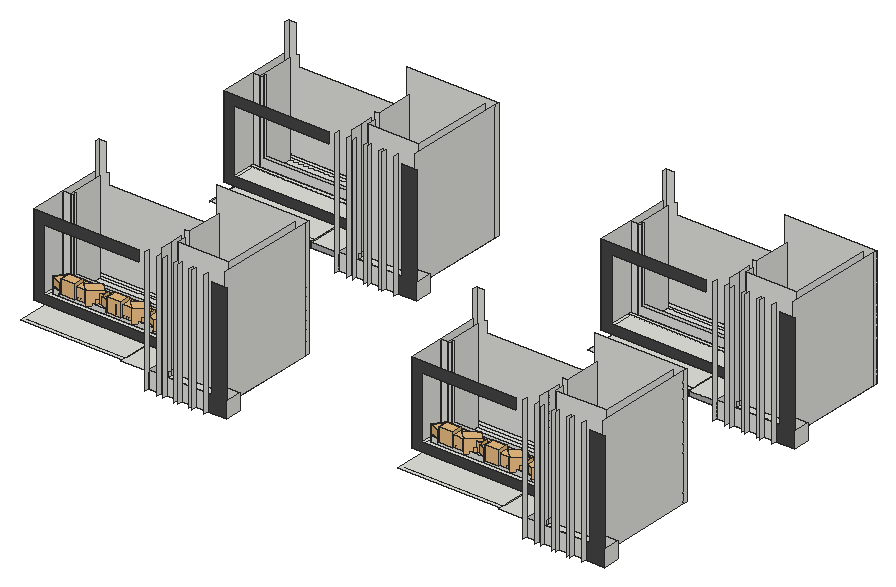
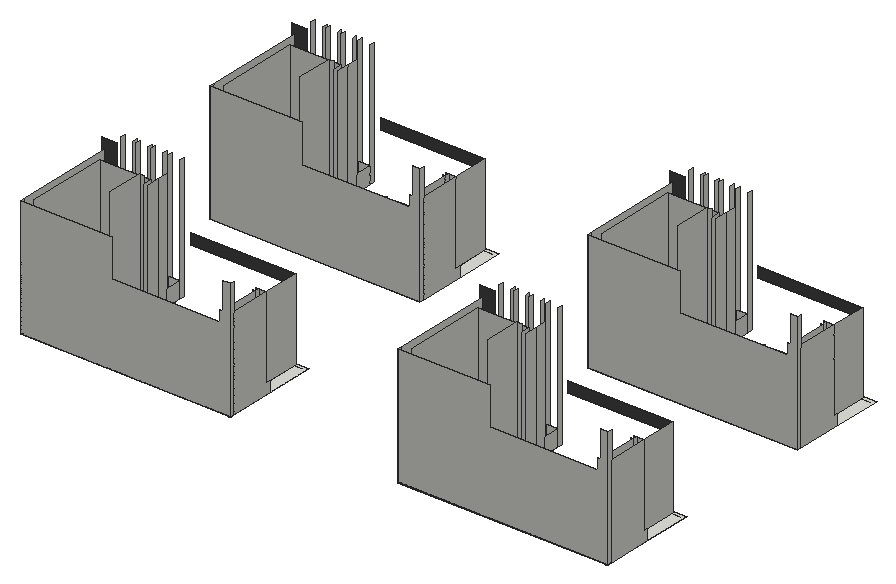
# SketchUp Ruby script. Lengths in inches.
U = 1.inch
M = Sketchup.active_model
def pt(a) = Geom::Point3d.new(a.map { |v| v * U })
def face(e, loops, mat)
  f = e.add_face(loops[0].map { |a| pt(a) })
  loops[1..].each { |l| e.add_face(l.map { |a| pt(a) }).erase! }
  f.material = f.back_material = mat if mat
  f
end
# faces: each face lists its corners as indices into pts; further lists are holes
def faces(e, pts, list, mat = nil) = list.each { |f| face(e, (f[0].is_a?(Array) ? f : [f]).map { |l| l.map { |i| pts[i] } }, mat) }
# xy, xz, yz: faces in a plane at the given z, y or x. An outline is a flat list of corners, or four numbers for a rectangle; further outlines are holes
def ring(l) = l.size == 4 ? [[l[0], l[1]], [l[2], l[1]], [l[2], l[3]], [l[0], l[3]]] : l.each_slice(2).to_a
def flat(e, list, mat, &to3) = list.each { |f| face(e, (f[0].is_a?(Array) ? f : [f]).map { |l| ring(l).map { |u, v| to3.(u, v) } }, mat) }
def xy(e, z, list, mat = nil) = flat(e, list, mat) { |x, y| [x, y, z] }
def xz(e, y, list, mat = nil) = flat(e, list, mat) { |x, z| [x, y, z] }
def yz(e, x, list, mat = nil) = flat(e, list, mat) { |y, z| [x, y, z] }
def lines(e, pts, list) = list.each { |a, b| e.add_line(pt(pts[a]), pt(pts[b])) }
# prism: a flat outline (further loops are holes) pulled along v
def prism(e, loops, v, mat = nil)
  f = face(e, loops, mat); d = Geom::Vector3d.new(v.map { |x| x * U })
  f.pushpull(f.normal.samedirection?(d) ? d.length : -d.length)
end
def box(e, o, s, mat = nil) = prism(e, [[o, [o[0] + s[0], o[1], o[2]], [o[0] + s[0], o[1] + s[1], o[2]], [o[0], o[1] + s[1], o[2]]]], [0, 0, s[2]], mat)
def at(x, y, z, deg = 0) = Geom::Transformation.translation(pt([x, y, z])) * Geom::Transformation.rotation(ORIGIN, Z_AXIS, deg.degrees)
def axes(o, x, y, z) = Geom::Transformation.new([*x, 0, *y, 0, *z, 0, *pt(o).to_a, 1])
def part(name) = M.definitions.add(name)
# library, detail: a bought-in or finely detailed component or shape, given as its bounding box
def library(name, o, s) = part(name).tap { |d| box(d.entities, o, s) }
def detail(e, o, s) = box(e.add_group.entities, o, s)
def put(e, d, t, mat = nil) = e.add_instance(d, t).tap { |i| i.material = mat if mat }
def group(e, t, mat = nil) = e.add_group.tap { |g| g.transformation = t; g.material = mat if mat }.entities
root = M.entities
M.materials.add("Material__1").color = [95, 70, 46]
M.materials.add("[Color M03]1").color = [170, 170, 170]
M.materials.add("[Granite Dark Gray]").color = [69, 68, 68]
c1 = library("Areca palm plant",[0,0,0],[49.1,36.6,54.46])
c2 = library("Group\#589",[-84.69,-90.07,-0.36],[176.51,175.13,171.4])
c3 = library("Group20\#1",[-20.81,-17.08,3.79],[39.86,39.43,37.51])
c4 = library("Group38\#1",[14.01,28.44,-23.43],[18.58,18.32,38.89])
c5 = library("Group\#590",[-7.34,-1.2,0],[38.67,35.81,49.04])
c6 = part("Group\#592")
put(c6.entities,c1,axes([-6.2,56.6,6.08],[0.45017,-0.56191,0],[0.66137,0.52986,0],[0,0,0.72]))
put(c6.entities,c1,axes([-6.2,158.41,6.08],[0.45017,-0.56191,0],[0.66137,0.52986,0],[0,0,0.72]))
put(c6.entities,c2,axes([17.19,15.79,6.07],[-0.08133,-0.14087,0],[0.14087,-0.08133,0],[0,0,0.1725]))
put(c6.entities,c3,axes([18.97,79.98,4.77],[0,0.85,0],[-0.85,0,0],[0,0,0.85]))
put(c6.entities,c4,axes([-4.1,-1.15,28.17],[0.8848,0,0],[0,0.94674,0],[0,0,0.85826]))
put(c6.entities,c2,axes([17.19,121.23,6.07],[-0.08133,-0.14087,0],[0.14087,-0.08133,0],[0,0,0.1725]))
put(c6.entities,c2,axes([14.93,91.37,6.05],[-0.04961,-0.08593,0],[0.08593,-0.04961,0],[0,0,0.10522]))
put(c6.entities,c3,axes([18.97,181.79,4.77],[0,0.85,0],[-0.85,0,0],[0,0,0.85]))
put(c6.entities,c2,axes([14.93,193.18,6.05],[-0.04961,-0.08593,0],[0.08593,-0.04961,0],[0,0,0.10522]))
put(c6.entities,c4,axes([-4.1,100.66,28.17],[0.8848,0,0],[0,0.94674,0],[0,0,0.85826]))
g1 = group(c6.entities,at(0,0,0))
xy(g1,0,[[0,0,6,234.8],[30,0,36,234.8]])
xy(g1,3,[[6,0,30,234.8]])
xy(g1,7,[[6,5,30,229.8]],"Material__1")
xy(g1,15,[[[0,0,36,234.8],[6,5,30,229.8]]])
xz(g1,0,[[0,0,6,0,6,3,30,3,30,0,36,0,36,15,0,15]])
xz(g1,5,[[6,7,30,15]])
xz(g1,229.8,[[6,7,30,15]])
xz(g1,234.8,[[0,0,0,15,36,15,36,0,30,0,30,3,6,3,6,0]])
yz(g1,0,[[0,0,234.8,15]])
yz(g1,6,[[0,0,234.8,3],[5,7,229.8,15]])
yz(g1,30,[[0,0,234.8,3],[5,7,229.8,15]])
yz(g1,36,[[0,0,234.8,15]])
put(c6.entities,c2,axes([17.19,223.04,6.07],[-0.08133,-0.14087,0],[0.14087,-0.08133,0],[0,0,0.1725]))
put(c6.entities,c2,axes([14.93,44.05,6.05],[-0.04961,-0.08593,0],[0.08593,-0.04961,0],[0,0,0.10522]))
put(c6.entities,c2,axes([14.93,173.12,6.05],[-0.04961,-0.08593,0],[0.08593,-0.04961,0],[0,0,0.10522]))
put(c6.entities,c2,axes([14.93,145.87,6.05],[-0.04961,-0.08593,0],[0.08593,-0.04961,0],[0,0,0.10522]))
put(c6.entities,c5,axes([24.9375,89.91,8],[0,0.79,0],[-0.79,0,0],[0,0,0.79]))
put(c6.entities,c2,axes([14.93,71.3,6.05],[-0.04961,-0.08593,0],[0.08593,-0.04961,0],[0,0,0.10522]))
put(c6.entities,c5,axes([24.9375,191.72,8],[0,0.79,0],[-0.79,0,0],[0,0,0.79]))
xy(root,144.9375,[[609.34,322.97,609.34,341.03,626.68,341.03,626.68,368.59,641.55,368.59,641.55,322.97],[641.55,322.97,657.03,387.84],[657.03,322.97,689.24,368.59],[689.24,322.97,698.65,387.84],[698.65,322.97,730.86,368.59],
  [730.86,322.97,739.28,387.84],[739.28,322.97,771.49,368.59],[771.49,322.97,771.49,387.84,782.78,387.84,782.78,368.59,824.53,368.59,824.53,322.97],[1657.65,322.97,1657.65,341.03,1674.99,341.03,1674.99,368.59,1689.86,368.59,1689.86,322.97],[1689.86,322.97,1705.34,387.84],
  [1705.34,322.97,1737.55,368.59],[1737.55,322.97,1746.96,387.84],[1746.96,322.97,1779.17,368.59],[1779.17,322.97,1787.59,387.84],[1787.59,322.97,1819.8,368.59],
  [1819.8,322.97,1819.8,387.84,1831.09,387.84,1831.09,368.59,1872.84,368.59,1872.84,322.97],[609.09,341.03,609.34,365.47],[609.34,341.03,626.68,365.47],[1657.41,341.03,1657.65,365.47],[1657.65,341.03,1674.99,365.47],
  [609.09,365.47,609.34,387.84],[609.34,365.47,626.68,368.59],[1657.41,365.47,1657.65,387.84],[1657.65,365.47,1674.99,368.59],[609.34,368.59,626.68,387.84],
  [626.68,368.59,641.55,387.84],[657.03,368.59,689.24,387.84],[698.65,368.59,730.86,387.84],[739.28,368.59,771.49,387.84],[1657.65,368.59,1674.99,387.84],
  [1674.99,368.59,1689.86,387.84],[1705.34,368.59,1737.55,387.84],[1746.96,368.59,1779.17,387.84],[1787.59,368.59,1819.8,387.84],[200.03,387.84,497.6,523.47],
  [[626.68,387.84,626.68,389.4,609.34,389.4,609.34,523.47,200.03,523.47,200.03,647.98,782.78,647.98,782.78,387.84],[620.86,408.96,761.66,408.96,761.66,637.97,221.15,637.97,221.15,534.98,620.86,534.98]],[609.09,387.84,609.34,389.4],[609.34,387.84,626.68,389.4],[1248.34,387.84,1545.92,523.47],[[1674.99,387.84,1674.99,389.4,1657.65,389.4,1657.65,523.47,1248.34,523.47,1248.34,647.98,1831.09,647.98,1831.09,387.84],[1669.17,408.96,1809.97,408.96,1809.97,637.97,1269.46,637.97,1269.46,534.98,1669.17,534.98]],
  [1657.41,387.84,1657.65,389.4],[1657.65,387.84,1674.99,389.4],[620.86,408.96,761.66,408.96,761.66,637.97,221.15,637.97,221.15,534.98,620.86,534.98],[1669.17,408.96,1809.97,408.96,1809.97,637.97,1269.46,637.97,1269.46,534.98,1669.17,534.98],[200.03,647.98,782.78,659.09],
  [1248.34,647.98,1831.09,659.09]])
xy(root,148.75,[[497.26,1024.56,497.26,1046.93,499.1875,1046.93,499.1875,1136.18,608.75,1136.18,608.75,1024.56],[608.75,1024.56,626.34,1046.93],[1545.57,1024.56,1545.57,1046.93,1547.5,1046.93,1547.5,1136.18,1657.0625,1136.18,1657.0625,1024.56],[1657.0625,1024.56,1674.65,1046.93],[608.75,1046.93,626.34,1046.93,626.34,1054,616.11,1054,616.11,1136.18,608.75,1136.18],
  [1657.0625,1046.93,1674.65,1046.93,1674.65,1054,1664.42,1054,1664.42,1136.18,1657.0625,1136.18],[616.11,1054,626.34,1136.18],[1664.42,1054,1674.65,1136.18],[607.28,1136.18,616.11,1153.68],[1655.6,1136.18,1664.42,1153.68]])
xy(root,149.375,[[609,982.06,609,1000.12,626.34,1000.12,626.34,1027.68,641.2,1027.68,641.2,982.06],[641.2,982.06,656.68,1046.93],[656.68,982.06,688.89,1027.68],[688.89,982.06,698.31,1046.93],[698.31,982.06,730.52,1027.68],
  [730.52,982.06,738.93,1046.93],[738.93,982.06,771.14,1027.68],[771.14,982.06,771.14,1046.93,782.4375,1046.93,782.4375,1027.68,824.1875,1027.68,824.1875,982.06],[1657.31,982.06,1657.31,1000.12,1674.65,1000.12,1674.65,1027.68,1689.52,1027.68,1689.52,982.06],[1689.52,982.06,1705,1046.93],
  [1705,982.06,1737.2,1027.68],[1737.2,982.06,1746.62,1046.93],[1746.62,982.06,1778.83,1027.68],[1778.83,982.06,1787.25,1046.93],[1787.25,982.06,1819.45,1027.68],
  [1819.45,982.06,1819.45,1046.93,1830.75,1046.93,1830.75,1027.68,1872.5,1027.68,1872.5,982.06],[608.75,1000.12,609,1024.56],[609,1000.12,626.34,1024.56],[1657.0625,1000.12,1657.31,1024.56],[1657.31,1000.12,1674.65,1024.56],
  [608.75,1024.56,609,1046.93],[609,1024.56,626.34,1027.68],[1657.0625,1024.56,1657.31,1046.93],[1657.31,1024.56,1674.65,1027.68],[609,1027.68,626.34,1046.93],
  [626.34,1027.68,641.2,1046.93],[656.68,1027.68,688.89,1046.93],[698.31,1027.68,730.52,1046.93],[738.93,1027.68,771.14,1046.93],[1657.31,1027.68,1674.65,1046.93],
  [1674.65,1027.68,1689.52,1046.93],[1705,1027.68,1737.2,1046.93],[1746.62,1027.68,1778.83,1046.93],[1787.25,1027.68,1819.45,1046.93],[199.6875,1046.93,497.26,1182.56],
  [[626.34,1046.93,626.34,1048.49,609,1048.49,609,1182.56,199.6875,1182.56,199.6875,1307.07,782.4375,1307.07,782.4375,1046.93],[620.51,1068.05,761.32,1068.05,761.32,1297.06,220.81,1297.06,220.81,1194.07,620.51,1194.07]],[608.75,1046.93,609,1048.49],[609,1046.93,626.34,1048.49],[1248,1046.93,1545.57,1182.56],[[1674.65,1046.93,1674.65,1048.49,1657.31,1048.49,1657.31,1182.56,1248,1182.56,1248,1307.07,1830.75,1307.07,1830.75,1046.93],[1668.82,1068.05,1809.63,1068.05,1809.63,1297.06,1269.12,1297.06,1269.12,1194.07,1668.82,1194.07]],
  [1657.0625,1046.93,1657.31,1048.49],[1657.31,1046.93,1674.65,1048.49],[620.51,1068.05,761.32,1068.05,761.32,1297.06,220.81,1297.06,220.81,1194.07,620.51,1194.07],[1668.82,1068.05,1809.63,1068.05,1809.63,1297.06,1269.12,1297.06,1269.12,1194.07,1668.82,1194.07],[199.6875,1307.07,782.4375,1318.18],
  [1248,1307.07,1830.75,1318.18]])
xy(root,157.5,[[497.6,365.47,609.09,365.47,609.09,387.84,609.34,387.84,609.34,523.47,497.6,523.47],[1545.92,365.47,1657.41,365.47,1657.41,387.84,1657.65,387.84,1657.65,523.47,1545.92,523.47]])
xy(root,161.9375,[[497.26,1024.56,608.75,1024.56,608.75,1046.93,609,1046.93,609,1182.56,497.26,1182.56],[1545.57,1024.56,1657.0625,1024.56,1657.0625,1046.93,1657.31,1046.93,1657.31,1182.56,1545.57,1182.56]])
xy(root,174.125,[[200.03,433.78,209.64,523.47],[609.34,433.78,609.34,523.47,200.03,523.47,200.03,534.98,620.86,534.98,620.86,433.78],[209.64,433.78,609.34,523.47],[620.86,433.78,632.79,534.98],[1248.34,433.78,1257.95,523.47],
  [1657.65,433.78,1657.65,523.47,1248.34,523.47,1248.34,534.98,1669.17,534.98,1669.17,433.78],[1257.95,433.78,1657.65,523.47],[1669.17,433.78,1681.11,534.98],[221.15,534.98,620.86,546.92],[620.86,534.98,632.79,546.92],
  [1269.46,534.98,1669.17,546.92],[1669.17,534.98,1681.11,546.92]])
xy(root,178.5625,[[199.6875,1092.87,209.29,1182.56],[609,1092.87,609,1182.56,199.6875,1182.56,199.6875,1194.07,620.51,1194.07,620.51,1092.87],[209.29,1092.87,609,1182.56],[620.51,1092.87,632.45,1194.07],[1248,1092.87,1257.61,1182.56],
  [1657.31,1092.87,1657.31,1182.56,1248,1182.56,1248,1194.07,1668.82,1194.07,1668.82,1092.87],[1257.61,1092.87,1657.31,1182.56],[1668.82,1092.87,1680.76,1194.07],[220.81,1194.07,620.51,1206.01],[620.51,1194.07,632.45,1206.01],
  [1269.12,1194.07,1668.82,1206.01],[1668.82,1194.07,1680.76,1206.01]])
xz(root,322.97,[[609.34,144.9375,641.55,191.19],[657.03,144.9375,689.24,191.19],[698.65,144.9375,730.86,191.19],[739.28,144.9375,771.49,191.19],[1657.65,144.9375,1689.86,191.19],
  [1705.34,144.9375,1737.55,191.19],[1746.96,144.9375,1779.17,191.19],[1787.59,144.9375,1819.8,191.19]])
xz(root,322.97,[[641.55,144.9375,657.03,191.19],[689.24,144.9375,698.65,191.19],[730.86,144.9375,739.28,191.19],[771.49,144.9375,824.53,144.9375,824.53,471.94,782.78,471.94,782.78,191.19,771.49,191.19],[1689.86,144.9375,1705.34,191.19],
  [1737.55,144.9375,1746.96,191.19],[1779.17,144.9375,1787.59,191.19],[1819.8,144.9375,1872.84,144.9375,1872.84,471.94,1831.09,471.94,1831.09,191.19,1819.8,191.19]],"[Granite Dark Gray]")
xz(root,368.59,[[782.78,144.9375,824.53,191.19],[1831.09,144.9375,1872.84,191.19]])
xz(root,387.84,[[609.09,144.9375,609.34,157.5],[1657.41,144.9375,1657.65,157.5]])
xz(root,408.96,[[620.86,144.9375,761.66,475.57],[1669.17,144.9375,1809.97,475.57]])
xz(root,433.78,[[609.34,174.125,620.86,199],[620.86,174.125,632.79,496.07],[1657.65,174.125,1669.17,199],[1669.17,174.125,1681.11,496.07]])
xz(root,433.78,[[200.03,174.125,609.34,174.125,609.34,199,228.06,199,228.06,370.64,490.99,370.64,490.99,400,200.03,400],[1248.34,174.125,1657.65,174.125,1657.65,199,1276.37,199,1276.37,370.64,1539.31,370.64,1539.31,400,1248.34,400]],"[Granite Dark Gray]")
xz(root,523.47,[[497.6,144.9375,609.34,157.5],[1545.92,144.9375,1657.65,157.5]])
xz(root,523.47,[[200.03,144.9375,497.6,144.9375,497.6,157.5,609.34,157.5,609.34,174.125,200.03,174.125],[1248.34,144.9375,1545.92,144.9375,1545.92,157.5,1657.65,157.5,1657.65,174.125,1248.34,174.125]],"[Color M03]1")
xz(root,534.98,[[221.15,144.9375,620.86,174.125],[1269.46,144.9375,1669.17,174.125],[200.03,174.125,221.15,400],[221.15,174.125,620.86,174.125,620.86,199,228.06,199,228.06,400,221.15,400],[620.86,174.125,632.79,199],
  [1248.34,174.125,1269.46,400],[1269.46,174.125,1669.17,174.125,1669.17,199,1276.37,199,1276.37,400,1269.46,400],[1669.17,174.125,1681.11,199]])
xz(root,546.92,[[221.15,174.125,221.15,400,228.06,400,228.06,199,620.86,199,620.86,174.125],[620.86,174.125,632.79,199],[1269.46,174.125,1269.46,400,1276.37,400,1276.37,199,1669.17,199,1669.17,174.125],[1669.17,174.125,1681.11,199]])
xz(root,659.09,[[200.03,144.9375,200.03,475.57,221.15,475.57,221.15,400,228.06,400,228.06,370.64,528.37,370.64,528.37,475.57,782.78,475.57,782.78,144.9375],[1248.34,144.9375,1248.34,475.57,1269.46,475.57,1269.46,400,1276.37,400,1276.37,370.64,1576.68,370.64,1576.68,475.57,1831.09,475.57,1831.09,144.9375]])
xz(root,982.06,[[609,149.375,641.2,195.63],[656.68,149.375,688.89,195.63],[698.31,149.375,730.52,195.63],[738.93,149.375,771.14,195.63],[1657.31,149.375,1689.52,195.63],
  [1705,149.375,1737.2,195.63],[1746.62,149.375,1778.83,195.63],[1787.25,149.375,1819.45,195.63]])
xz(root,982.06,[[641.2,149.375,656.68,195.63],[688.89,149.375,698.31,195.63],[730.52,149.375,738.93,195.63],[771.14,149.375,824.1875,149.375,824.1875,476.38,782.4375,476.38,782.4375,195.63,771.14,195.63],[1689.52,149.375,1705,195.63],
  [1737.2,149.375,1746.62,195.63],[1778.83,149.375,1787.25,195.63],[1819.45,149.375,1872.5,149.375,1872.5,476.38,1830.75,476.38,1830.75,195.63,1819.45,195.63]],"[Granite Dark Gray]")
xz(root,1024.56,[[608.75,148.75,626.34,149.375],[1657.0625,148.75,1674.65,149.375]])
xz(root,1024.56,[[497.26,148.75,608.75,161.9375],[1545.57,148.75,1657.0625,161.9375]],"[Color M03]1")
xz(root,1027.68,[[782.4375,149.375,824.1875,195.63],[1830.75,149.375,1872.5,195.63]])
xz(root,1046.93,[[608.75,148.75,609,149.375],[609,148.75,626.34,149.375],[626.34,148.75,641.2,149.375],[641.2,148.75,656.68,149.375],[688.89,148.75,698.31,149.375],
  [730.52,148.75,738.93,149.375],[771.14,148.75,782.4375,149.375],[1657.0625,148.75,1657.31,149.375],[1657.31,148.75,1674.65,149.375],[1674.65,148.75,1689.52,149.375],
  [1689.52,148.75,1705,149.375],[1737.2,148.75,1746.62,149.375],[1778.83,148.75,1787.25,149.375],[1819.45,148.75,1830.75,149.375],[608.75,149.375,609,161.9375],
  [1657.0625,149.375,1657.31,161.9375]])
xz(root,1068.05,[[620.51,149.375,761.32,480],[1668.82,149.375,1809.63,480]])
xz(root,1092.87,[[609,178.5625,620.51,203.4375],[620.51,178.5625,632.45,500.5],[1657.31,178.5625,1668.82,203.4375],[1668.82,178.5625,1680.76,500.5]])
xz(root,1092.87,[[199.6875,178.5625,609,178.5625,609,203.4375,227.71,203.4375,227.71,375.08,490.65,375.08,490.65,404.4375,199.6875,404.4375],[1248,178.5625,1657.31,178.5625,1657.31,203.4375,1276.02,203.4375,1276.02,375.08,1538.96,375.08,1538.96,404.4375,1248,404.4375]],"[Granite Dark Gray]")
xz(root,1182.56,[[497.26,149.375,609,161.9375],[1545.57,149.375,1657.31,161.9375]])
xz(root,1182.56,[[199.6875,149.375,497.26,149.375,497.26,161.9375,609,161.9375,609,178.5625,199.6875,178.5625],[1248,149.375,1545.57,149.375,1545.57,161.9375,1657.31,161.9375,1657.31,178.5625,1248,178.5625]],"[Color M03]1")
xz(root,1194.07,[[220.81,149.375,620.51,178.5625],[1269.12,149.375,1668.82,178.5625],[199.6875,178.5625,220.81,404.4375],[220.81,178.5625,620.51,178.5625,620.51,203.4375,227.71,203.4375,227.71,404.4375,220.81,404.4375],[620.51,178.5625,632.45,203.4375],
  [1248,178.5625,1269.12,404.4375],[1269.12,178.5625,1668.82,178.5625,1668.82,203.4375,1276.02,203.4375,1276.02,404.4375,1269.12,404.4375],[1668.82,178.5625,1680.76,203.4375]])
xz(root,1206.01,[[220.81,178.5625,220.81,404.4375,227.71,404.4375,227.71,203.4375,620.51,203.4375,620.51,178.5625],[620.51,178.5625,632.45,203.4375],[1269.12,178.5625,1269.12,404.4375,1276.02,404.4375,1276.02,203.4375,1668.82,203.4375,1668.82,178.5625],[1668.82,178.5625,1680.76,203.4375]])
xz(root,1318.18,[[199.6875,148.75,782.4375,149.375],[1248,148.75,1830.75,149.375],[199.6875,149.375,199.6875,480,220.81,480,220.81,404.4375,227.71,404.4375,227.71,375.08,528.02,375.08,528.02,480,782.4375,480,782.4375,149.375],[1248,149.375,1248,480,1269.12,480,1269.12,404.4375,1276.02,404.4375,1276.02,375.08,1576.34,375.08,1576.34,480,1830.75,480,1830.75,149.375]])
yz(root,199.6875,[[1046.93,148.75,1318.18,149.375],[1182.56,149.375,1182.56,178.5625,1194.07,178.5625,1194.07,404.4375,1307.07,404.4375,1307.07,149.375],[1307.07,149.375,1318.18,480],[1092.87,178.5625,1194.07,404.4375]])
yz(root,200.03,[[523.47,144.9375,523.47,174.125,534.98,174.125,534.98,400,647.98,400,647.98,144.9375],[647.98,144.9375,659.09,475.57],[433.78,174.125,534.98,400]])
yz(root,220.81,[[1194.07,149.375,1297.06,149.375,1297.06,404.4375,1206.01,404.4375,1206.01,178.5625,1194.07,178.5625],[1194.07,178.5625,1206.01,404.4375]])
yz(root,221.15,[[534.98,144.9375,637.97,144.9375,637.97,400,546.92,400,546.92,174.125,534.98,174.125],[534.98,174.125,546.92,400]])
yz(root,497.26,[[1024.56,148.75,1046.93,161.9375],[1046.93,149.375,1056.54,161.9375],[1056.54,149.375,1182.56,161.9375]])
yz(root,497.6,[[387.84,144.9375,397.45,157.5],[397.45,144.9375,523.47,157.5]])
yz(root,608.75,[[1024.56,148.75,1046.93,149.375],[1046.93,148.75,1048.49,149.375],[1024.56,149.375,1046.93,161.9375]])
yz(root,609,[[968.74,149.375,982.06,495.5],[982.06,149.375,1027.68,195.63],[1027.68,149.375,1027.68,480,1056.54,480,1056.54,161.9375,1046.93,161.9375,1046.93,149.375],[1046.93,149.375,1056.54,161.9375],[1056.54,149.375,1182.56,161.9375],
  [1056.54,161.9375,1056.54,480,1092.87,480,1092.87,178.5625,1182.56,178.5625,1182.56,161.9375]])
yz(root,609.09,[[365.47,144.9375,387.84,157.5]])
yz(root,609.34,[[309.65,144.9375,322.97,491.07],[322.97,144.9375,368.59,191.19],[368.59,144.9375,368.59,475.57,397.45,475.57,397.45,157.5,387.84,157.5,387.84,144.9375],[387.84,144.9375,397.45,157.5],[397.45,144.9375,523.47,157.5],
  [397.45,157.5,397.45,475.57,433.78,475.57,433.78,174.125,523.47,174.125,523.47,157.5]])
yz(root,620.51,[[1068.05,149.375,1194.07,149.375,1194.07,178.5625,1092.87,178.5625,1092.87,480,1068.05,480],[1092.87,178.5625,1194.07,203.4375],[1194.07,178.5625,1206.01,203.4375]])
yz(root,620.86,[[408.96,144.9375,534.98,144.9375,534.98,174.125,433.78,174.125,433.78,475.57,408.96,475.57],[433.78,174.125,534.98,199],[534.98,174.125,546.92,199]])
yz(root,626.34,[[1024.56,148.75,1046.93,149.375],[1046.93,148.75,1048.49,149.375]])
yz(root,632.45,[[1092.87,178.5625,1194.07,500.5],[1194.07,178.5625,1206.01,203.4375]])
yz(root,632.79,[[433.78,174.125,534.98,496.07],[534.98,174.125,546.92,199]])
yz(root,641.2,[[968.74,149.375,982.06,495.5]])
yz(root,641.55,[[309.65,144.9375,322.97,491.07]])
yz(root,656.68,[[968.74,149.375,982.06,495.5]])
yz(root,657.03,[[309.65,144.9375,322.97,491.07]])
yz(root,688.89,[[968.74,149.375,982.06,495.5]])
yz(root,689.24,[[309.65,144.9375,322.97,491.07]])
yz(root,698.31,[[968.74,149.375,982.06,495.5]])
yz(root,698.65,[[309.65,144.9375,322.97,491.07]])
yz(root,730.52,[[968.74,149.375,982.06,495.5]])
yz(root,730.86,[[309.65,144.9375,322.97,491.07]])
yz(root,738.93,[[968.74,149.375,982.06,495.5]])
yz(root,739.28,[[309.65,144.9375,322.97,491.07]])
yz(root,761.32,[[1068.05,149.375,1297.06,480]])
yz(root,761.66,[[408.96,144.9375,637.97,475.57]])
yz(root,771.14,[[968.74,149.375,982.06,495.5]])
yz(root,771.49,[[309.65,144.9375,322.97,491.07]])
yz(root,782.4375,[[1046.93,148.75,1318.18,149.375],[1027.68,149.375,1307.07,480],[1307.07,149.375,1318.18,480]])
yz(root,782.78,[[368.59,144.9375,647.98,475.57],[647.98,144.9375,659.09,475.57]])
yz(root,824.1875,[[982.06,149.375,1027.68,195.63]])
yz(root,824.53,[[322.97,144.9375,368.59,191.19]])
yz(root,1248,[[1046.93,148.75,1318.18,149.375],[1182.56,149.375,1182.56,178.5625,1194.07,178.5625,1194.07,404.4375,1307.07,404.4375,1307.07,149.375],[1307.07,149.375,1318.18,480],[1092.87,178.5625,1194.07,404.4375]])
yz(root,1248.34,[[523.47,144.9375,523.47,174.125,534.98,174.125,534.98,400,647.98,400,647.98,144.9375],[647.98,144.9375,659.09,475.57],[433.78,174.125,534.98,400]])
yz(root,1269.12,[[1194.07,149.375,1297.06,149.375,1297.06,404.4375,1206.01,404.4375,1206.01,178.5625,1194.07,178.5625],[1194.07,178.5625,1206.01,404.4375]])
yz(root,1269.46,[[534.98,144.9375,637.97,144.9375,637.97,400,546.92,400,546.92,174.125,534.98,174.125],[534.98,174.125,546.92,400]])
yz(root,1545.57,[[1024.56,148.75,1046.93,161.9375],[1046.93,149.375,1056.54,161.9375],[1056.54,149.375,1182.56,161.9375]])
yz(root,1545.92,[[387.84,144.9375,397.45,157.5],[397.45,144.9375,523.47,157.5]])
yz(root,1657.0625,[[1024.56,148.75,1046.93,149.375],[1046.93,148.75,1048.49,149.375],[1024.56,149.375,1046.93,161.9375]])
yz(root,1657.31,[[968.74,149.375,982.06,495.5],[982.06,149.375,1027.68,195.63],[1027.68,149.375,1027.68,480,1056.54,480,1056.54,161.9375,1046.93,161.9375,1046.93,149.375],[1046.93,149.375,1056.54,161.9375],[1056.54,149.375,1182.56,161.9375],
  [1056.54,161.9375,1056.54,480,1092.87,480,1092.87,178.5625,1182.56,178.5625,1182.56,161.9375]])
yz(root,1657.41,[[365.47,144.9375,387.84,157.5]])
yz(root,1657.65,[[309.65,144.9375,322.97,491.07],[322.97,144.9375,368.59,191.19],[368.59,144.9375,368.59,475.57,397.45,475.57,397.45,157.5,387.84,157.5,387.84,144.9375],[387.84,144.9375,397.45,157.5],[397.45,144.9375,523.47,157.5],
  [397.45,157.5,397.45,475.57,433.78,475.57,433.78,174.125,523.47,174.125,523.47,157.5]])
yz(root,1668.82,[[1068.05,149.375,1194.07,149.375,1194.07,178.5625,1092.87,178.5625,1092.87,480,1068.05,480],[1092.87,178.5625,1194.07,203.4375],[1194.07,178.5625,1206.01,203.4375]])
yz(root,1669.17,[[408.96,144.9375,534.98,144.9375,534.98,174.125,433.78,174.125,433.78,475.57,408.96,475.57],[433.78,174.125,534.98,199],[534.98,174.125,546.92,199]])
yz(root,1674.65,[[1024.56,148.75,1046.93,149.375],[1046.93,148.75,1048.49,149.375]])
yz(root,1680.76,[[1092.87,178.5625,1194.07,500.5],[1194.07,178.5625,1206.01,203.4375]])
yz(root,1681.11,[[433.78,174.125,534.98,496.07],[534.98,174.125,546.92,199]])
yz(root,1689.52,[[968.74,149.375,982.06,495.5]])
yz(root,1689.86,[[309.65,144.9375,322.97,491.07]])
yz(root,1705,[[968.74,149.375,982.06,495.5]])
yz(root,1705.34,[[309.65,144.9375,322.97,491.07]])
yz(root,1737.2,[[968.74,149.375,982.06,495.5]])
yz(root,1737.55,[[309.65,144.9375,322.97,491.07]])
yz(root,1746.62,[[968.74,149.375,982.06,495.5]])
yz(root,1746.96,[[309.65,144.9375,322.97,491.07]])
yz(root,1778.83,[[968.74,149.375,982.06,495.5]])
yz(root,1779.17,[[309.65,144.9375,322.97,491.07]])
yz(root,1787.25,[[968.74,149.375,982.06,495.5]])
yz(root,1787.59,[[309.65,144.9375,322.97,491.07]])
yz(root,1809.63,[[1068.05,149.375,1297.06,480]])
yz(root,1809.97,[[408.96,144.9375,637.97,475.57]])
yz(root,1819.45,[[968.74,149.375,982.06,495.5]])
yz(root,1819.8,[[309.65,144.9375,322.97,491.07]])
yz(root,1830.75,[[1046.93,148.75,1318.18,149.375],[1027.68,149.375,1307.07,480],[1307.07,149.375,1318.18,480]])
yz(root,1831.09,[[368.59,144.9375,647.98,475.57],[647.98,144.9375,659.09,475.57]])
yz(root,1872.5,[[982.06,149.375,1027.68,195.63]])
yz(root,1872.84,[[322.97,144.9375,368.59,191.19]])
p = [[209.64,397.45,144.9375],[497.6,397.45,144.9375],[1257.95,397.45,144.9375],[1545.92,397.45,144.9375],[209.29,1056.54,149.375],[497.26,1056.54,149.375],
  [208.57,1054,148.75],[208.57,1046.93,148.75],[497.26,1054,148.75],[497.26,1046.93,148.75],[1257.61,1056.54,149.375],[1545.57,1056.54,149.375],
  [1256.88,1054,148.75],[1256.88,1046.93,148.75],[1545.57,1054,148.75],[1545.57,1046.93,148.75]]
lines(root,p,[[0,1],[2,3],[4,5],[6,7],[8,9],[10,11],[12,13],[14,15]])
put(root,c6,axes([524.375,465.95,184.9375],[0,1,0],[-1.25931,0,0],[0,0,1]))
put(root,c6,axes([1572.6875,465.95,184.9375],[0,1,0],[-1.25931,0,0],[0,0,1]))
